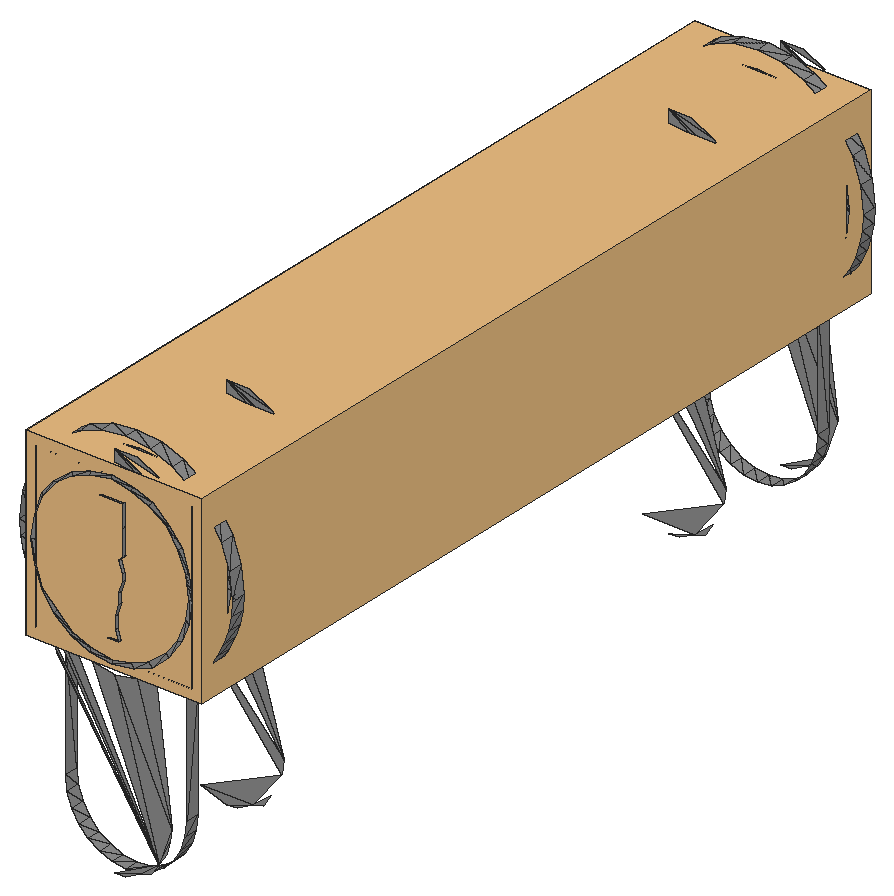
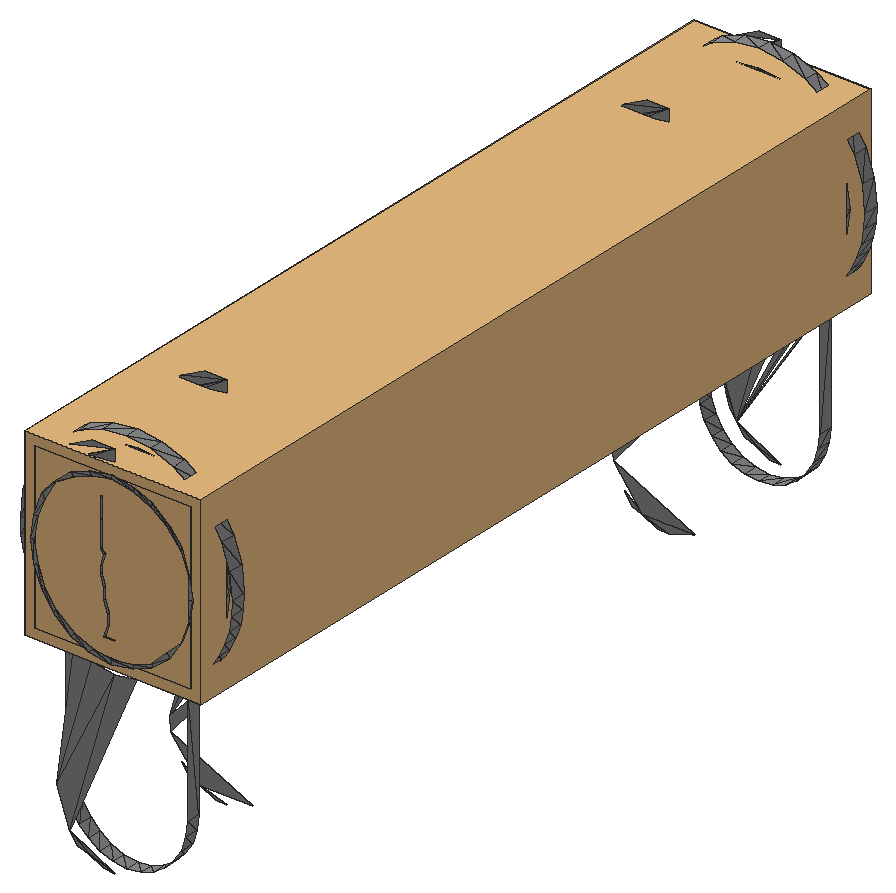
# SketchUp Ruby script. Lengths in inches.
U = 1.inch
M = Sketchup.active_model
def pt(a) = Geom::Point3d.new(a.map { |v| v * U })
def face(e, loops, mat)
  f = e.add_face(loops[0].map { |a| pt(a) })
  loops[1..].each { |l| e.add_face(l.map { |a| pt(a) }).erase! }
  f.material = f.back_material = mat if mat
  f
end
# faces: each face lists its corners as indices into pts; further lists are holes
def faces(e, pts, list, mat = nil) = list.each { |f| face(e, (f[0].is_a?(Array) ? f : [f]).map { |l| l.map { |i| pts[i] } }, mat) }
# xy, xz, yz: faces in a plane at the given z, y or x. An outline is a flat list of corners, or four numbers for a rectangle; further outlines are holes
def ring(l) = l.size == 4 ? [[l[0], l[1]], [l[2], l[1]], [l[2], l[3]], [l[0], l[3]]] : l.each_slice(2).to_a
def flat(e, list, mat, &to3) = list.each { |f| face(e, (f[0].is_a?(Array) ? f : [f]).map { |l| ring(l).map { |u, v| to3.(u, v) } }, mat) }
def xy(e, z, list, mat = nil) = flat(e, list, mat) { |x, y| [x, y, z] }
def xz(e, y, list, mat = nil) = flat(e, list, mat) { |x, z| [x, y, z] }
def yz(e, x, list, mat = nil) = flat(e, list, mat) { |y, z| [x, y, z] }
def lines(e, pts, list) = list.each { |a, b| e.add_line(pt(pts[a]), pt(pts[b])) }
# prism: a flat outline (further loops are holes) pulled along v
def prism(e, loops, v, mat = nil)
  f = face(e, loops, mat); d = Geom::Vector3d.new(v.map { |x| x * U })
  f.pushpull(f.normal.samedirection?(d) ? d.length : -d.length)
end
def box(e, o, s, mat = nil) = prism(e, [[o, [o[0] + s[0], o[1], o[2]], [o[0] + s[0], o[1] + s[1], o[2]], [o[0], o[1] + s[1], o[2]]]], [0, 0, s[2]], mat)
def at(x, y, z, deg = 0) = Geom::Transformation.translation(pt([x, y, z])) * Geom::Transformation.rotation(ORIGIN, Z_AXIS, deg.degrees)
def axes(o, x, y, z) = Geom::Transformation.new([*x, 0, *y, 0, *z, 0, *pt(o).to_a, 1])
def part(name) = M.definitions.add(name)
# library, detail: a bought-in or finely detailed component or shape, given as its bounding box
def library(name, o, s) = part(name).tap { |d| box(d.entities, o, s) }
def detail(e, o, s) = box(e.add_group.entities, o, s)
def put(e, d, t, mat = nil) = e.add_instance(d, t).tap { |i| i.material = mat if mat }
def group(e, t, mat = nil) = e.add_group.tap { |g| g.transformation = t; g.material = mat if mat }.entities
root = M.entities
M.materials.add("Material \#1").color = [140, 140, 140]
c1 = library("3DGeom~12_Defintion",[-95.68,-755.75,-830.03],[191.36,191.37,1000])
c2 = part("3DGeom~10_Defintion")
yz(c2.entities,-68.96,[[-797.08,-844.83,-797.08,-827.59,-922.41,-827.59],[-922.41,-844.83,-797.08,-844.83,-922.41,-827.59]],"Material \#1")
yz(c2.entities,68.97,[[-922.41,-844.83,-797.08,-827.59,-797.08,-844.83],[-922.41,-844.83,-922.41,-827.59,-797.08,-827.59],[-797.08,137.93,-922.41,155.17,-797.08,155.17],[-922.41,137.93,-922.41,155.17,-797.08,137.93]],"Material \#1")
p = [[-15.8,-989.55,-844.83],[-15.8,-989.55,-827.59],[0,-991.38,-827.59],[0,-991.38,-844.83],[15.8,-989.55,-827.59],[15.8,-989.55,-844.83],
  [-30.32,-984.36,-844.83],[-30.32,-984.36,-827.59],[30.31,-984.36,-827.59],[30.31,-984.36,-844.83],[-43.12,-976.21,-844.83],[-43.12,-976.21,-827.59],
  [43.12,-976.21,-827.59],[43.12,-976.21,-844.83],[-53.81,-965.53,-844.83],[-53.81,-965.53,-827.59],[53.8,-965.53,-827.59],[53.8,-965.53,-844.83],
  [-61.95,-952.73,-844.83],[-61.95,-952.73,-827.59],[53.8,-965.53,-827.59],[61.95,-952.73,-827.59],[61.95,-952.73,-844.83],[-67.15,-938.21,-844.83],
  [-67.15,-938.21,-827.59],[67.14,-938.21,-827.59],[67.14,-938.21,-844.83],[-68.96,-922.41,-844.83],[-68.96,-922.41,-827.59],[67.14,-938.21,-827.59],
  [68.97,-922.41,-827.59],[68.97,-922.41,-844.83],[-69.1,-794.86,-844.83],[-69.1,-794.86,-827.59],[-68.96,-797.08,-827.59],[-68.96,-797.08,-844.83],
  [68.97,-797.08,-844.83],[68.97,-797.08,-827.59],[69.11,-794.71,-827.59],[69.11,-794.71,-844.83],[-69.48,-792.73,-844.83],[-69.48,-792.73,-827.59],
  [69.53,-792.51,-827.59],[69.53,-792.51,-844.83],[-70.14,-790.6875,-844.83],[-70.14,-790.6875,-827.59],[70.24,-790.48,-827.59],[70.24,-790.48,-844.83],
  [-71.08,-788.73,-844.83],[-71.08,-788.73,-827.59],[71.22,-788.57,-827.59],[71.22,-788.57,-844.83],[-72.32,-786.86,-844.83],[-72.32,-786.86,-827.59],
  [72.47,-786.78,-827.59],[72.47,-786.78,-844.83],[-73.8,-785.17,-844.83],[-73.8,-785.17,-827.59],[74,-785.04,-827.59],[74,-785.04,-844.83],
  [-75.96,-783.21,-844.83],[-75.96,-783.21,-827.59],[74,-785.04,-827.59],[75.76,-783.39,-827.59],[75.76,-783.39,-844.83],[86.625,-772.95,-827.59],
  [86.61,-772.96,-844.83],[-86.89,-773.25,-844.83],[-86.89,-773.25,-827.59],[-75.96,-783.21,-844.83],[-96.66,-761.8,-844.83],[-96.66,-761.8,-827.59],
  [86.625,-772.95,-827.59],[86.63,-772.94,-844.83],[86.61,-772.96,-844.83],[86.625,-772.95,-827.59],[86.62,-772.95,-827.59],[86.62,-772.95,-827.59],
  [96.31,-761.375,-827.59],[96.31,-761.375,-844.83],[86.63,-772.94,-844.83],[86.625,-772.95,-827.59],[86.62,-772.95,-827.59],[-104.96,-749.18,-844.83],
  [-104.96,-749.18,-827.59],[-96.66,-761.8,-827.59],[-96.66,-761.8,-844.83],[96.31,-761.375,-827.59],[104.62,-748.77,-827.59],[104.62,-748.77,-844.83],
  [-111.64,-735.52,-844.83],[-111.64,-735.52,-827.59],[111.39,-735.21,-827.59],[111.39,-735.21,-844.83],[-116.49,-721.23,-844.83],[-116.49,-721.23,-827.59],
  [116.4375,-720.78,-827.59],[116.4375,-720.78,-844.83],[-119.64,-705.62,-844.83],[-119.64,-705.62,-827.59],[119.6,-705.57,-827.59],[119.6,-705.57,-844.83],
  [-120.6875,-689.65,-844.83],[-120.6875,-689.65,-827.59],[120.69,-689.65,-827.59],[120.69,-689.65,-844.83],[-117.5,-662,-844.83],[-117.5,-662,-827.59],
  [117.5,-662,-827.59],[117.5,-662,-844.83],[-108.41,-636.61,-844.83],[-108.41,-636.61,-827.59],[117.5,-662,-844.83],[108.41,-636.61,-827.59],
  [108.41,-636.61,-844.83],[-93.91,-613.95,-844.83],[-93.91,-613.95,-827.59],[-108.41,-636.61,-827.59],[108.41,-636.61,-844.83],[94.16,-614.19,-827.59],
  [94.16,-614.19,-844.83],[94.16,-614.19,-827.59],[75.46,-595.5,-827.59],[75.46,-595.5,-844.83],[-75.46,-595.5,-844.83],[-75.46,-595.5,-827.59],
  [-93.91,-613.95,-827.59],[-93.91,-613.95,-827.59],[-93.91,-613.95,-844.83],[-53.05,-581.24,-844.83],[-53.05,-581.24,-827.59],[-75.46,-595.5,-827.59],
  [-75.46,-595.5,-844.83],[53.05,-581.24,-827.59],[53.05,-581.24,-844.83],[-27.65,-572.16,-844.83],[-27.65,-572.16,-827.59],[-53.05,-581.24,-827.59],
  [-53.05,-581.24,-844.83],[27.66,-572.16,-827.59],[27.66,-572.16,-844.83],[0,-568.97,-844.83],[0,-568.97,-827.59],[-27.65,-572.16,-827.59],
  [-27.65,-572.16,-844.83],[0,-568.97,-844.83],[-15.8,-989.55,155.17],[0,-991.38,155.17],[0,-991.38,137.93],[-15.8,-989.55,137.93],
  [15.8,-989.55,155.17],[15.8,-989.55,137.93],[-30.32,-984.36,155.17],[-30.32,-984.36,137.93],[30.31,-984.36,155.17],[30.31,-984.36,137.93],
  [-43.125,-976.22,155.17],[-43.125,-976.22,137.93],[43.12,-976.22,155.17],[43.12,-976.22,137.93],[-53.81,-965.53,155.17],[-53.81,-965.53,137.93],
  [53.8,-965.53,155.17],[53.8,-965.53,137.93],[-61.96,-952.73,155.17],[-61.95,-952.73,137.93],[61.95,-952.73,155.17],[61.95,-952.73,137.93],
  [53.8,-965.53,137.93],[-67.15,-938.21,155.17],[-67.15,-938.21,137.93],[67.14,-938.21,155.17],[67.14,-938.21,137.93],[-68.96,-922.41,155.17],
  [-68.96,-922.41,137.93],[68.97,-922.41,155.17],[68.97,-922.41,137.93],[67.14,-938.21,137.93],[-68.97,-797.08,155.17],[-68.97,-797.08,137.93],
  [-69.1,-794.86,155.17],[-69.1,-794.86,137.93],[68.97,-797.08,155.17],[69.11,-794.71,155.17],[69.11,-794.71,137.93],[68.97,-797.08,137.93],
  [-69.48,-792.73,155.17],[-69.48,-792.73,137.93],[69.53,-792.51,155.17],[69.53,-792.51,137.93],[-70.14,-790.6875,155.17],[-70.14,-790.6875,137.93],
  [70.24,-790.48,155.17],[70.24,-790.48,137.93],[-71.08,-788.73,155.17],[-71.08,-788.73,137.93],[71.22,-788.57,155.17],[71.22,-788.57,137.93],
  [-72.32,-786.86,155.17],[-72.32,-786.86,137.93],[72.47,-786.78,155.17],[72.47,-786.78,137.93],[-73.8,-785.17,155.17],[-73.8,-785.17,137.93],
  [74,-785.04,155.17],[74,-785.04,137.93],[-75.96,-783.21,155.17],[-75.96,-783.21,137.93],[75.76,-783.39,155.17],[75.76,-783.39,137.93],
  [74,-785.04,137.93],[86.61,-772.96,155.17],[86.625,-772.95,137.93],[-86.88,-773.25,155.17],[-75.96,-783.21,155.17],[-86.88,-773.25,137.93],
  [-96.66,-761.8,155.17],[-96.66,-761.8,137.93],[86.63,-772.94,155.17],[86.625,-772.95,137.93],[86.61,-772.96,155.17],[86.62,-772.95,137.93],
  [86.625,-772.95,137.93],[96.31,-761.375,155.17],[96.31,-761.375,137.93],[86.62,-772.95,137.93],[86.63,-772.94,155.17],[86.62,-772.95,137.93],
  [86.625,-772.95,137.93],[-104.96,-749.18,155.17],[-96.66,-761.8,155.17],[-96.66,-761.8,137.93],[-104.96,-749.18,137.93],[104.62,-748.77,155.17],
  [104.62,-748.77,137.93],[96.31,-761.375,137.93],[-111.64,-735.52,155.17],[-111.64,-735.52,137.93],[111.39,-735.21,155.17],[111.39,-735.21,137.93],
  [-116.49,-721.23,155.17],[-116.49,-721.23,137.93],[116.4375,-720.78,155.17],[116.4375,-720.78,137.93],[-119.64,-705.62,155.17],[-119.64,-705.62,137.93],
  [119.6,-705.57,155.17],[119.6,-705.57,137.93],[-120.6875,-689.65,155.17],[-120.6875,-689.65,137.93],[120.69,-689.65,155.17],[120.69,-689.65,137.93],
  [-117.5,-662,155.17],[-117.5,-662,137.93],[117.5,-662,155.17],[117.5,-662,137.93],[-108.41,-636.61,155.17],[-108.41,-636.61,137.93],
  [117.5,-662,155.17],[108.41,-636.61,155.17],[108.41,-636.61,137.93],[-93.91,-613.95,155.17],[-108.41,-636.61,137.93],[-93.91,-613.95,137.93],
  [108.41,-636.61,155.17],[94.16,-614.19,155.17],[94.16,-614.19,137.93],[75.46,-595.5,155.17],[75.46,-595.5,137.93],[94.16,-614.19,137.93],
  [-75.46,-595.5,155.17],[-93.91,-613.95,155.17],[-93.91,-613.95,137.93],[-75.46,-595.5,137.93],[-53.05,-581.24,155.17],[-75.46,-595.5,155.17],
  [-75.46,-595.5,137.93],[-53.05,-581.24,137.93],[53.05,-581.24,155.17],[53.05,-581.24,137.93],[-27.65,-572.16,155.17],[-53.05,-581.24,155.17],
  [-53.05,-581.24,137.93],[-27.65,-572.16,137.93],[27.65,-572.16,155.17],[27.65,-572.16,137.93],[0,-568.97,155.17],[-27.65,-572.16,155.17],
  [-27.65,-572.16,137.93],[0,-568.97,137.93],[0,-568.97,155.17]]
faces(c2.entities,p,[[0,1,2],[2,3,0],[3,2,4],[4,5,3],[6,7,1],[1,0,6],[5,4,8],[8,9,5],
  [10,11,7],[7,6,10],[9,8,12],[12,13,9],[14,15,11],[11,10,14],[13,12,16],[16,17,13],
  [18,19,15],[15,14,18],[17,20,21],[21,22,17],[23,24,19],[19,18,23],[22,21,25],[25,26,22],
  [27,28,24],[24,23,27],[26,29,30],[30,31,26],[32,33,34],[34,35,32],[36,37,38],[38,39,36],
  [40,41,33],[33,32,40],[39,38,42],[42,43,39],[44,45,41],[41,40,44],[43,42,46],[46,47,43],
  [48,49,45],[45,44,48],[47,46,50],[50,51,47],[52,53,49],[49,48,52],[51,50,54],[54,55,51],
  [56,57,53],[53,52,56],[55,54,58],[58,59,55],[60,61,57],[57,56,60],[59,62,63],[63,64,59],
  [64,63,65],[65,66,64],[67,68,61],[61,69,67],[70,71,68],[68,67,70],[72,73,66],[74,75,76],
  [73,77,78],[78,79,73],[80,81,82],[83,84,85],[85,86,83],[79,87,88],[88,89,79],[90,91,84],
  [84,83,90],[89,88,92],[92,93,89],[94,95,91],[91,90,94],[93,92,96],[96,97,93],[98,99,95],
  [95,94,98],[97,96,100],[100,101,97],[102,103,99],[99,98,102],[101,100,104],[104,105,101],[106,107,103],
  [103,102,106],[105,104,108],[108,109,105],[110,111,107],[107,106,110],[112,108,113],[113,114,112],[115,116,117],
  [117,110,115],[118,113,119],[119,120,118],[120,121,122],[122,123,120],[124,125,126],[127,128,124],[129,130,131],
  [131,132,129],[123,122,133],[133,134,123],[135,136,137],[137,138,135],[134,133,139],[139,140,134],[141,142,143],
  [143,144,141],[140,139,142],[142,145,140],[146,147,148],[148,149,146],[147,150,151],[151,148,147],[152,146,149],
  [149,153,152],[150,154,155],[155,151,150],[156,152,153],[153,157,156],[154,158,159],[159,155,154],[160,156,157],
  [157,161,160],[158,162,163],[163,159,158],[164,160,161],[161,165,164],[162,166,167],[167,168,162],[169,164,165],
  [165,170,169],[166,171,172],[172,167,166],[173,169,170],[170,174,173],[171,175,176],[176,177,171],[178,173,174],
  [174,179,178],[180,178,179],[179,181,180],[182,183,184],[184,185,182],[186,180,181],[181,187,186],[183,188,189],
  [189,184,183],[190,186,187],[187,191,190],[188,192,193],[193,189,188],[194,190,191],[191,195,194],[192,196,197],
  [197,193,192],[198,194,195],[195,199,198],[196,200,201],[201,197,196],[202,198,199],[199,203,202],[200,204,205],
  [205,201,200],[206,202,203],[203,207,206],[204,208,209],[209,210,204],[208,211,212],[212,209,208],[213,214,207],
  [207,215,213],[216,213,215],[215,217,216],[211,218,219],[220,221,222],[218,223,224],[224,225,218],[226,227,228],
  [229,230,231],[231,232,229],[223,233,234],[234,235,223],[236,229,232],[232,237,236],[233,238,239],[239,234,233],
  [240,236,237],[237,241,240],[238,242,243],[243,239,238],[244,240,241],[241,245,244],[242,246,247],[247,243,242],
  [248,244,245],[245,249,248],[246,250,251],[251,247,246],[252,248,249],[249,253,252],[250,254,255],[255,251,250],
  [256,252,253],[253,257,256],[258,259,260],[260,255,258],[261,256,262],[262,263,261],[264,265,266],[266,260,264],
  [265,267,268],[268,269,265],[270,271,272],[272,273,270],[274,275,276],[276,277,274],[267,278,279],[279,268,267],
  [280,281,282],[282,283,280],[278,284,285],[285,279,278],[286,287,288],[288,289,286],[284,290,289],[289,285,284]],"Material \#1")
c3 = library("3DGeom~13_Defintion",[-84.91,-744.98,-830.03],[169.82,169.83,1000])
xy(root,30.51,[[337.207,116.513,337.207,116.862,337.243,116.862],[337.207,116.513,337.243,116.862,337.243,116.513],[337.207,118.4375,337.207,118.786,337.243,118.4375],[337.243,118.4375,337.207,118.786,337.243,118.786]],"Material \#1")
xy(root,30.853,[[337.189,116.513,337.249,116.513,337.189,116.862],[337.249,116.513,337.249,116.862,337.189,116.862],[337.189,118.4375,337.249,118.4375,337.249,118.786]],"Material \#1")
xz(root,116.513,[[337.219,30.452,337.162,30.46,337.219,30.46],[337.219,30.452,337.219,30.46,337.274,30.468],[337.219,30.452,337.274,30.468,337.276,30.46],[337.162,30.46,337.108,30.482,337.164,30.468],[337.162,30.46,337.164,30.468,337.219,30.46],
  [337.276,30.46,337.274,30.468,337.325,30.49],[337.276,30.46,337.325,30.49,337.329,30.482],[337.164,30.468,337.108,30.482,337.112,30.49],[337.108,30.482,337.0625,30.519,337.112,30.49],[337.329,30.482,337.325,30.49,337.369,30.525],
  [337.329,30.482,337.369,30.525,337.375,30.519],[337.112,30.49,337.0625,30.519,337.068,30.525],[337.0625,30.519,337.028,30.567,337.068,30.525],[337.375,30.519,337.369,30.525,337.402,30.571],[337.375,30.519,337.402,30.571,337.41,30.567],
  [337.068,30.525,337.028,30.567,337.035,30.571],[337.028,30.567,337.005,30.622,337.035,30.571],[337.41,30.567,337.402,30.571,337.424,30.624],[337.41,30.567,337.424,30.624,337.432,30.622],[337.035,30.571,337.005,30.622,337.014,30.624],
  [337.005,30.622,336.998,30.681,337.014,30.624],[337.432,30.622,337.424,30.624,337.431,30.681],[337.432,30.622,337.431,30.681,337.439,30.681],[337.014,30.624,336.998,30.681,337.006,30.681],[336.998,30.681,337.005,30.741,337.006,30.681],
  [337.006,30.681,337.005,30.741,337.014,30.738],[337.431,30.681,337.424,30.738,337.439,30.681],[337.439,30.681,337.424,30.738,337.432,30.741],[337.014,30.738,337.005,30.741,337.028,30.796],[337.014,30.738,337.028,30.796,337.035,30.792],
  [337.424,30.738,337.402,30.792,337.432,30.741],[337.432,30.741,337.402,30.792,337.41,30.796],[337.035,30.792,337.028,30.796,337.0625,30.844],[337.035,30.792,337.0625,30.844,337.068,30.838],[337.402,30.792,337.369,30.838,337.41,30.796],
  [337.41,30.796,337.369,30.838,337.375,30.844],[337.068,30.838,337.0625,30.844,337.108,30.88],[337.068,30.838,337.108,30.88,337.112,30.873],[337.369,30.838,337.325,30.873,337.375,30.844],[337.375,30.844,337.325,30.873,337.329,30.88],
  [337.112,30.873,337.108,30.88,337.162,30.903],[337.112,30.873,337.162,30.903,337.164,30.895],[337.325,30.873,337.274,30.895,337.329,30.88],[337.329,30.88,337.274,30.895,337.276,30.903],[337.164,30.895,337.162,30.903,337.219,30.911],
  [337.164,30.895,337.219,30.911,337.219,30.902],[337.274,30.895,337.219,30.902,337.276,30.903],[337.219,30.902,337.219,30.911,337.276,30.903]],"Material \#1")
xz(root,116.525,[[337.219,29.939,337.288,29.955,337.255,29.943],[337.219,29.939,337.341,30,337.288,29.955],[337.288,29.955,337.341,30,337.317,29.974],[337.341,30,337.025,30.52,337.064,30.48],[337.341,30,337.058,30.433,337.056,30.439],
  [337.341,30,337.06,30.427,337.058,30.433],[337.341,30,337.061,30.42,337.06,30.427],[337.341,30,337.064,30.48,337.11,30.45],[337.341,30,337.162,30.431,337.219,30.424],[337.341,30,337.219,30.424,337.375,30.102],
  [337.341,30,337.371,30.064,337.359,30.03],[337.341,30,337.375,30.102,337.371,30.064],[337.375,30.102,337.219,30.424,337.275,30.431],[337.375,30.102,337.275,30.431,337.327,30.45],[337.4375,30.864,337.327,30.913,337.219,30.973],
  [337.327,30.913,337.275,30.932,337.219,30.973],[337.275,30.932,337.219,30.939,337.219,30.973],[337.342,30.944,337.219,30.973,337.283,30.966]],"Material \#1")
xz(root,116.6,[[337.219,30.424,337.155,30.432,337.219,30.432],[337.219,30.424,337.219,30.432,337.281,30.441],[337.219,30.424,337.281,30.441,337.283,30.432],[337.155,30.432,337.095,30.458,337.157,30.441],[337.155,30.432,337.157,30.441,337.219,30.432],
  [337.283,30.432,337.281,30.441,337.338,30.466],[337.283,30.432,337.338,30.466,337.342,30.458],[337.157,30.441,337.095,30.458,337.099,30.466],[337.095,30.458,337.044,30.499,337.099,30.466],[337.342,30.458,337.338,30.466,337.388,30.505],
  [337.342,30.458,337.388,30.505,337.394,30.499],[337.099,30.466,337.044,30.499,337.049,30.505],[337.044,30.499,337.004,30.553,337.049,30.505],[337.394,30.499,337.388,30.505,337.426,30.557],[337.394,30.499,337.426,30.557,337.433,30.553],
  [337.049,30.505,337.004,30.553,337.011,30.557],[337.004,30.553,336.979,30.615,337.011,30.557],[337.433,30.553,337.426,30.557,337.45,30.617],[337.433,30.553,337.45,30.617,337.458,30.615],[337.011,30.557,336.979,30.615,336.988,30.617],
  [336.979,30.615,336.971,30.681,336.988,30.617],[337.458,30.615,337.45,30.617,337.458,30.681],[337.458,30.615,337.458,30.681,337.466,30.681],[336.988,30.617,336.971,30.681,336.979,30.681],[336.971,30.681,336.979,30.748,336.979,30.681],
  [336.979,30.681,336.979,30.748,336.988,30.746],[337.458,30.681,337.45,30.746,337.466,30.681],[337.466,30.681,337.45,30.746,337.458,30.748],[336.988,30.746,336.979,30.748,337.004,30.81],[336.988,30.746,337.004,30.81,337.011,30.806],
  [337.45,30.746,337.426,30.806,337.458,30.748],[337.458,30.748,337.426,30.806,337.433,30.81],[337.011,30.806,337.004,30.81,337.044,30.863],[337.011,30.806,337.044,30.863,337.049,30.857],[337.426,30.806,337.388,30.857,337.433,30.81],
  [337.433,30.81,337.388,30.857,337.394,30.863],[337.049,30.857,337.044,30.863,337.095,30.904],[337.049,30.857,337.095,30.904,337.099,30.897],[337.388,30.857,337.338,30.897,337.394,30.863],[337.394,30.863,337.338,30.897,337.342,30.904],
  [337.099,30.897,337.095,30.904,337.155,30.93],[337.099,30.897,337.155,30.93,337.157,30.922],[337.338,30.897,337.281,30.922,337.342,30.904],[337.342,30.904,337.281,30.922,337.283,30.93],[337.157,30.922,337.155,30.93,337.219,30.939],
  [337.157,30.922,337.219,30.939,337.219,30.93],[337.281,30.922,337.219,30.93,337.283,30.93],[337.219,30.93,337.219,30.939,337.283,30.93]],"Material \#1")
xz(root,116.9,[[337.219,29.939,337.288,29.955,337.15,29.955],[337.219,29.939,337.255,29.943,337.288,29.955],[337.15,29.955,337.288,29.955,337.371,30.064],[337.288,29.955,337.317,29.974,337.341,30],[337.371,30.064,337.375,30.102,337.056,30.439],
  [337.375,30.102,337.219,30.424,337.162,30.431],[337.375,30.102,337.275,30.431,337.219,30.424],[337.275,30.431,337.382,30.439,337.327,30.45],[337.4375,30.864,337.219,30.973,337.327,30.913],[337.4375,30.864,337.342,30.944,337.219,30.973],
  [337.327,30.913,337.219,30.973,337.275,30.932],[337.275,30.932,337.219,30.973,337.219,30.939],[337.342,30.944,337.283,30.966,337.219,30.973]],"Material \#1")
xz(root,118.4,[[337.219,29.939,337.288,29.955,337.255,29.943],[337.15,29.955,337.371,30.064,337.288,29.955],[337.288,29.955,337.341,30,337.317,29.974],[337.371,30.064,337.056,30.439,337.375,30.102],[337.375,30.102,337.162,30.431,337.219,30.424],
  [337.375,30.102,337.219,30.424,337.275,30.431],[337.275,30.431,337.327,30.45,337.382,30.439],[337.4375,30.864,337.219,30.973,337.342,30.944],[337.4375,30.864,337.327,30.913,337.219,30.973],[337.327,30.913,337.275,30.932,337.219,30.973],
  [337.275,30.932,337.219,30.939,337.219,30.973],[337.342,30.944,337.219,30.973,337.283,30.966]],"Material \#1")
xz(root,118.7,[[337.219,30.424,337.219,30.432,337.155,30.432],[337.219,30.424,337.281,30.441,337.219,30.432],[337.219,30.424,337.283,30.432,337.281,30.441],[337.155,30.432,337.157,30.441,337.095,30.458],[337.155,30.432,337.219,30.432,337.157,30.441],
  [337.283,30.432,337.338,30.466,337.281,30.441],[337.283,30.432,337.342,30.458,337.338,30.466],[337.157,30.441,337.099,30.466,337.095,30.458],[337.095,30.458,337.099,30.466,337.044,30.499],[337.342,30.458,337.388,30.505,337.338,30.466],
  [337.342,30.458,337.394,30.499,337.388,30.505],[337.099,30.466,337.049,30.505,337.044,30.499],[337.044,30.499,337.049,30.505,337.004,30.553],[337.394,30.499,337.426,30.557,337.388,30.505],[337.394,30.499,337.433,30.553,337.426,30.557],
  [337.049,30.505,337.011,30.557,337.004,30.553],[337.004,30.553,337.011,30.557,336.979,30.615],[337.433,30.553,337.45,30.617,337.426,30.557],[337.433,30.553,337.458,30.615,337.45,30.617],[337.011,30.557,336.988,30.617,336.979,30.615],
  [336.979,30.615,336.988,30.617,336.971,30.681],[337.458,30.615,337.458,30.681,337.45,30.617],[337.458,30.615,337.466,30.681,337.458,30.681],[336.988,30.617,336.979,30.681,336.971,30.681],[336.971,30.681,336.979,30.681,336.979,30.748],
  [336.979,30.681,336.988,30.746,336.979,30.748],[337.458,30.681,337.466,30.681,337.45,30.746],[337.466,30.681,337.458,30.748,337.45,30.746],[336.988,30.746,337.004,30.81,336.979,30.748],[336.988,30.746,337.011,30.806,337.004,30.81],
  [337.45,30.746,337.458,30.748,337.426,30.806],[337.458,30.748,337.433,30.81,337.426,30.806],[337.011,30.806,337.044,30.863,337.004,30.81],[337.011,30.806,337.049,30.857,337.044,30.863],[337.426,30.806,337.433,30.81,337.388,30.857],
  [337.433,30.81,337.394,30.863,337.388,30.857],[337.049,30.857,337.095,30.904,337.044,30.863],[337.049,30.857,337.099,30.897,337.095,30.904],[337.388,30.857,337.394,30.863,337.338,30.897],[337.394,30.863,337.342,30.904,337.338,30.897],
  [337.099,30.897,337.155,30.93,337.095,30.904],[337.099,30.897,337.157,30.922,337.155,30.93],[337.338,30.897,337.342,30.904,337.281,30.922],[337.342,30.904,337.283,30.93,337.281,30.922],[337.157,30.922,337.219,30.939,337.155,30.93],
  [337.157,30.922,337.219,30.93,337.219,30.939],[337.281,30.922,337.283,30.93,337.219,30.93],[337.219,30.93,337.283,30.93,337.219,30.939]],"Material \#1")
xz(root,118.775,[[337.219,29.939,337.255,29.943,337.288,29.955],[337.219,29.939,337.288,29.955,337.341,30],[337.288,29.955,337.317,29.974,337.341,30],[337.341,30,337.219,30.424,337.162,30.431],[337.341,30,337.375,30.102,337.219,30.424],
  [337.375,30.102,337.275,30.431,337.219,30.424],[337.375,30.102,337.327,30.45,337.275,30.431],[337.4375,30.864,337.219,30.973,337.327,30.913],[337.327,30.913,337.219,30.973,337.275,30.932],[337.275,30.932,337.219,30.973,337.219,30.939],
  [337.342,30.944,337.283,30.966,337.219,30.973]],"Material \#1")
xz(root,118.786,[[337.219,30.452,337.219,30.46,337.162,30.46],[337.219,30.452,337.274,30.468,337.219,30.46],[337.219,30.452,337.276,30.46,337.274,30.468],[337.162,30.46,337.164,30.468,337.108,30.482],[337.162,30.46,337.219,30.46,337.164,30.468],
  [337.276,30.46,337.325,30.49,337.274,30.468],[337.276,30.46,337.329,30.482,337.325,30.49],[337.164,30.468,337.112,30.49,337.108,30.482],[337.108,30.482,337.112,30.49,337.0625,30.519],[337.329,30.482,337.369,30.525,337.325,30.49],
  [337.329,30.482,337.375,30.519,337.369,30.525],[337.112,30.49,337.068,30.525,337.0625,30.519],[337.0625,30.519,337.068,30.525,337.028,30.567],[337.375,30.519,337.402,30.571,337.369,30.525],[337.375,30.519,337.41,30.567,337.402,30.571],
  [337.068,30.525,337.035,30.571,337.028,30.567],[337.028,30.567,337.035,30.571,337.005,30.622],[337.41,30.567,337.424,30.624,337.402,30.571],[337.41,30.567,337.432,30.622,337.424,30.624],[337.035,30.571,337.014,30.624,337.005,30.622],
  [337.005,30.622,337.014,30.624,336.998,30.681],[337.432,30.622,337.431,30.681,337.424,30.624],[337.432,30.622,337.439,30.681,337.431,30.681],[337.014,30.624,337.006,30.681,336.998,30.681],[336.998,30.681,337.006,30.681,337.005,30.741],
  [337.006,30.681,337.014,30.738,337.005,30.741],[337.431,30.681,337.439,30.681,337.424,30.738],[337.439,30.681,337.432,30.741,337.424,30.738],[337.014,30.738,337.028,30.796,337.005,30.741],[337.014,30.738,337.035,30.792,337.028,30.796],
  [337.424,30.738,337.432,30.741,337.402,30.792],[337.432,30.741,337.41,30.796,337.402,30.792],[337.035,30.792,337.0625,30.844,337.028,30.796],[337.035,30.792,337.068,30.838,337.0625,30.844],[337.402,30.792,337.41,30.796,337.369,30.838],
  [337.41,30.796,337.375,30.844,337.369,30.838],[337.068,30.838,337.108,30.88,337.0625,30.844],[337.068,30.838,337.112,30.873,337.108,30.88],[337.369,30.838,337.375,30.844,337.325,30.873],[337.375,30.844,337.329,30.88,337.325,30.873],
  [337.112,30.873,337.162,30.903,337.108,30.88],[337.112,30.873,337.164,30.895,337.162,30.903],[337.325,30.873,337.329,30.88,337.274,30.895],[337.329,30.88,337.276,30.903,337.274,30.895],[337.164,30.895,337.219,30.911,337.162,30.903],
  [337.164,30.895,337.219,30.902,337.219,30.911],[337.274,30.895,337.276,30.903,337.219,30.902],[337.219,30.902,337.276,30.903,337.219,30.911]],"Material \#1")
yz(root,337.243,[[116.513,30.604,116.862,30.604,116.862,30.634],[116.513,30.604,116.862,30.634,116.513,30.634],[118.4375,30.604,118.786,30.604,118.4375,30.634],[118.786,30.604,118.786,30.634,118.4375,30.634]],"Material \#1")
yz(root,337.249,[[116.513,30.724,116.862,30.724,116.862,30.78],[118.4375,30.724,118.786,30.724,118.4375,30.78]],"Material \#1")
yz(root,337.252,[[116.513,30.658,116.862,30.658,116.862,30.683],[116.513,30.658,116.862,30.683,116.513,30.683],[118.4375,30.658,118.786,30.658,118.4375,30.683],[118.786,30.658,118.786,30.683,118.4375,30.683]],"Material \#1")
p = [[337.234,116.513,30.54],[337.231,116.862,30.535],[337.237,116.862,30.544],[337.234,116.513,30.54],[337.237,116.862,30.544],[337.237,116.862,30.563],
  [337.234,116.513,30.568],[337.231,116.862,30.535],[337.234,116.513,30.54],[337.243,116.513,30.51],[337.243,116.513,30.51],[337.243,116.862,30.51],
  [337.231,116.862,30.535],[337.234,118.786,30.54],[337.237,118.4375,30.544],[337.231,118.4375,30.535],[337.234,118.786,30.54],[337.234,118.786,30.568],
  [337.237,118.4375,30.563],[337.237,118.4375,30.544],[337.243,118.786,30.51],[337.234,118.786,30.54],[337.231,118.4375,30.535],[337.231,118.4375,30.535],
  [337.243,118.4375,30.51],[337.243,118.786,30.51],[337.234,116.513,30.568],[337.237,116.862,30.563],[337.231,116.862,30.572],[337.234,116.513,30.568],
  [337.231,116.862,30.572],[337.243,116.862,30.604],[337.243,116.862,30.604],[337.243,116.513,30.604],[337.234,116.513,30.568],[337.243,116.513,30.634],
  [337.243,116.862,30.634],[337.252,116.862,30.658],[337.252,116.862,30.658],[337.252,116.513,30.658],[337.243,116.513,30.634],[337.234,118.786,30.568],
  [337.231,118.4375,30.572],[337.237,118.4375,30.563],[337.243,118.4375,30.604],[337.231,118.4375,30.572],[337.234,118.786,30.568],[337.234,118.786,30.568],
  [337.243,118.786,30.604],[337.243,118.4375,30.604],[337.243,118.786,30.634],[337.252,118.786,30.658],[337.252,118.4375,30.658],[337.243,118.4375,30.634],
  [337.243,116.513,30.707],[337.243,116.862,30.707],[337.249,116.862,30.724],[337.243,116.862,30.707],[337.243,116.513,30.707],[337.252,116.513,30.683],
  [337.249,116.862,30.724],[337.249,116.513,30.724],[337.243,116.513,30.707],[337.249,116.862,30.78],[337.246,116.513,30.791],[337.249,116.513,30.724],
  [337.252,116.513,30.683],[337.252,116.862,30.683],[337.243,116.862,30.707],[337.249,118.4375,30.724],[337.243,118.4375,30.707],[337.243,118.786,30.707],
  [337.252,118.786,30.683],[337.243,118.786,30.707],[337.243,118.4375,30.707],[337.243,118.786,30.707],[337.249,118.786,30.724],[337.249,118.4375,30.724],
  [337.249,118.786,30.724],[337.246,118.786,30.791],[337.249,118.4375,30.78],[337.243,118.4375,30.707],[337.252,118.4375,30.683],[337.252,118.786,30.683],
  [337.246,116.513,30.791],[337.249,116.862,30.797],[337.249,116.862,30.853],[337.249,116.862,30.853],[337.249,116.513,30.853],[337.246,116.513,30.791],
  [337.249,118.4375,30.853],[337.249,118.4375,30.797],[337.246,118.786,30.791],[337.246,118.786,30.791],[337.249,118.786,30.853],[337.249,118.4375,30.853]]
faces(root,p,[[0,1,2],[3,4,5],[5,6,3],[7,8,9],[10,11,12],[13,14,15],[16,17,18],[18,19,16],
  [20,21,22],[23,24,25],[26,27,28],[29,30,31],[32,33,34],[35,36,37],[38,39,40],[41,42,43],
  [44,45,46],[47,48,49],[50,51,52],[52,53,50],[54,55,56],[57,58,59],[60,61,62],[63,64,65],
  [66,67,68],[69,70,71],[72,73,74],[75,76,77],[78,79,80],[81,82,83],[84,85,86],[87,88,89],
  [90,91,92],[93,94,95]],"Material \#1")
put(root,c1,axes([337.22,118.4,32.4],[0.0025,0,0],[0,0,0.0026],[0,0.00227,0]),"Material \#1")
put(root,c2,axes([337.22,118.4,32.4],[0.00239,0,0],[0,0,0.00249],[0,0.00218,0]),"Material \#1")
put(root,c3,axes([337.22,118.4,32.4],[0.0025,0,0],[0,0,0.0026],[0,0.00227,0]),"Material \#1")
